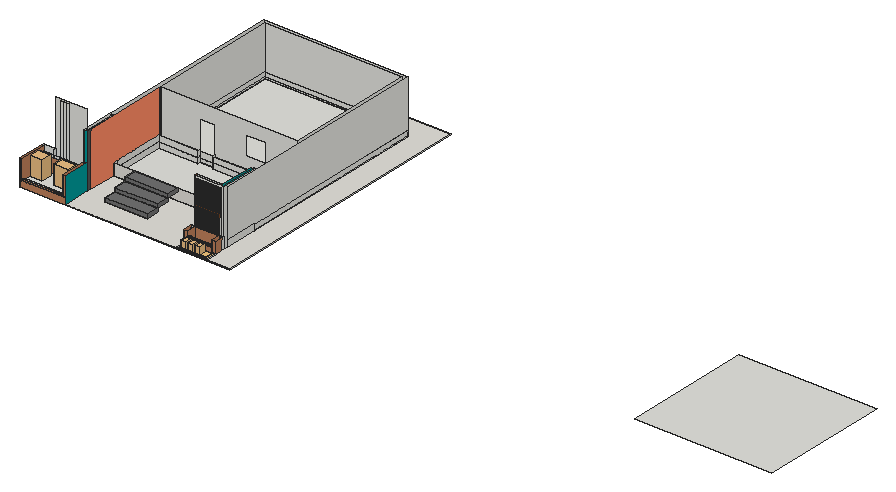
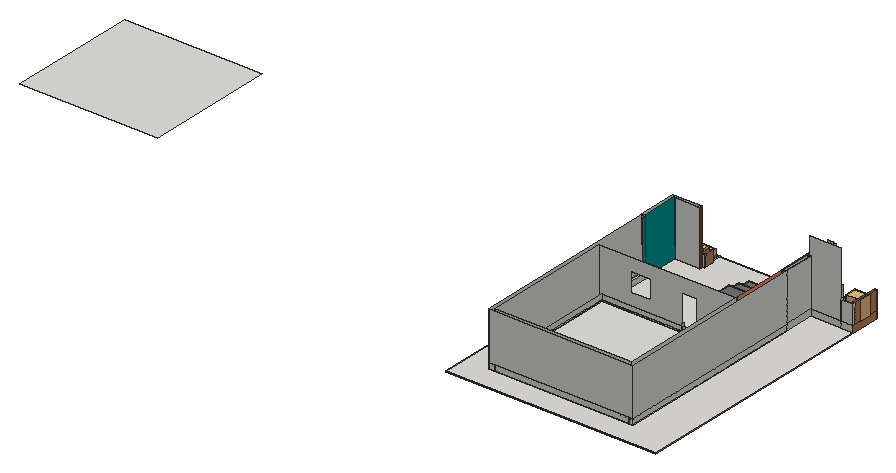
# SketchUp Ruby script. Lengths in inches.
U = 1.inch
M = Sketchup.active_model
def pt(a) = Geom::Point3d.new(a.map { |v| v * U })
def face(e, loops, mat)
  f = e.add_face(loops[0].map { |a| pt(a) })
  loops[1..].each { |l| e.add_face(l.map { |a| pt(a) }).erase! }
  f.material = f.back_material = mat if mat
  f
end
# faces: each face lists its corners as indices into pts; further lists are holes
def faces(e, pts, list, mat = nil) = list.each { |f| face(e, (f[0].is_a?(Array) ? f : [f]).map { |l| l.map { |i| pts[i] } }, mat) }
# xy, xz, yz: faces in a plane at the given z, y or x. An outline is a flat list of corners, or four numbers for a rectangle; further outlines are holes
def ring(l) = l.size == 4 ? [[l[0], l[1]], [l[2], l[1]], [l[2], l[3]], [l[0], l[3]]] : l.each_slice(2).to_a
def flat(e, list, mat, &to3) = list.each { |f| face(e, (f[0].is_a?(Array) ? f : [f]).map { |l| ring(l).map { |u, v| to3.(u, v) } }, mat) }
def xy(e, z, list, mat = nil) = flat(e, list, mat) { |x, y| [x, y, z] }
def xz(e, y, list, mat = nil) = flat(e, list, mat) { |x, z| [x, y, z] }
def yz(e, x, list, mat = nil) = flat(e, list, mat) { |y, z| [x, y, z] }
def lines(e, pts, list) = list.each { |a, b| e.add_line(pt(pts[a]), pt(pts[b])) }
# prism: a flat outline (further loops are holes) pulled along v
def prism(e, loops, v, mat = nil)
  f = face(e, loops, mat); d = Geom::Vector3d.new(v.map { |x| x * U })
  f.pushpull(f.normal.samedirection?(d) ? d.length : -d.length)
end
def box(e, o, s, mat = nil) = prism(e, [[o, [o[0] + s[0], o[1], o[2]], [o[0] + s[0], o[1] + s[1], o[2]], [o[0], o[1] + s[1], o[2]]]], [0, 0, s[2]], mat)
def at(x, y, z, deg = 0) = Geom::Transformation.translation(pt([x, y, z])) * Geom::Transformation.rotation(ORIGIN, Z_AXIS, deg.degrees)
def axes(o, x, y, z) = Geom::Transformation.new([*x, 0, *y, 0, *z, 0, *pt(o).to_a, 1])
def part(name) = M.definitions.add(name)
# library, detail: a bought-in or finely detailed component or shape, given as its bounding box
def library(name, o, s) = part(name).tap { |d| box(d.entities, o, s) }
def detail(e, o, s) = box(e.add_group.entities, o, s)
def put(e, d, t, mat = nil) = e.add_instance(d, t).tap { |i| i.material = mat if mat }
def group(e, t, mat = nil) = e.add_group.tap { |g| g.transformation = t; g.material = mat if mat }.entities
root = M.entities
M.materials.add("[Color B03]").color = [255, 140, 101]
M.materials.add("[Color H07]").color = [0, 153, 153]
M.materials.add("[Color M05]").color = [114, 114, 114]
M.materials.add("[Color M06]").color = [86, 86, 86]
M.materials.add("[Marble Carrara Gold Floor Tile]").color = [225, 223, 217]
M.materials.add("[Wood OSB]").color = [240, 195, 122]
M.materials.add("[Wood Veneer 01]").color = [120, 70, 37]
M.materials.add("[Wood Veneer 02]").color = [190, 128, 91]
c1 = library("Flower+vase",[-27.04,-0.0625,0],[7.8,7.11,11.89])
c2 = library("Decorative Plant",[-0.35,-0.24,0],[4.14,4.48,6.875])
xy(root,-18.75,[[114.76,294.58,448.89,619.58]])
xy(root,-14.75,[[[0,0,523.53,687.4],[104.7,148.58,464.7,628.58]]])
xy(root,-13.375,[[391.11,0,391.11,27.35,395.24,27.35,395.24,6.2,458.71,6.2,458.71,27.35,464.58,27.35,464.58,0],[386.33,27.35,395.89,48.85],[395.89,27.35,455.01,32.63],[455.01,27.35,464.58,48.85],[395.89,32.63,455.01,48.85],
  [386.33,48.85,464.58,53.1],[104.7,148.58,104.7,628.58,114.76,628.58,114.76,148.89,113.7,148.89,113.7,148.58],[113.7,148.58,114.76,148.89],[114.76,148.58,448.89,148.89],[448.89,148.58,455.7,148.89],
  [455.7,148.58,455.7,148.89,448.89,148.89,448.89,626.64,464.7,626.64,464.7,148.58],[448.89,626.64,464.7,628.58],[104.7,628.58,448.89,628.89]])
xy(root,-13.375,[[112.66,0,391.11,0,391.11,27.35,386.33,27.35,386.33,53.1,464.58,53.1,464.58,0,523.53,0,523.53,687.4,0,687.4,0,73.72,104.7,73.72,104.7,628.89,448.89,628.89,448.89,628.58,464.7,628.58,464.7,65.3,455.7,65.3,455.7,148.58,113.7,148.58,113.7,78.01,113.42,78.01,113.42,67.32,112.66,67.32]],"[Marble Carrara Gold Floor Tile]")
xy(root,-13.375,[[395.24,6.2,458.71,27.35]],"[Wood OSB]")
xy(root,-13.25,[[113.7,148.89,113.7,288.58,212.89,288.58,212.89,294.58,248.89,294.58,248.89,288.58,455.7,288.58,455.7,148.89]])
xy(root,-11.375,[[391.11,0,464.58,0,464.58,27.35,458.71,27.35,458.71,6.2,395.24,6.2,395.24,27.35,391.11,27.35]],"[Wood OSB]")
xy(root,-3.625,[[114.76,294.58,448.89,619.58]])
xy(root,-1.375,[[395.89,27.35,455.01,32.63]],"[Color M05]")
xy(root,0,[[1526.25,8.36,1868.25,333.36],[104.7,148.58,113.7,148.58,113.7,288.58,114.76,288.58,114.76,294.58,113.7,294.58,113.7,619.58,114.76,619.58,114.76,628.58,104.7,628.58],[113.7,148.58,114.76,288.58],[448.89,148.58,455.7,288.58],[455.7,148.58,464.7,148.58,464.7,626.64,448.89,626.64,448.89,619.58,455.7,619.58,455.7,294.58,448.89,294.58,448.89,288.58,455.7,288.58],
  [114.76,288.58,212.89,294.58],[248.89,288.58,448.89,294.58],[113.7,294.58,114.76,619.58],[448.89,294.58,455.7,619.58],[114.76,619.58,448.89,628.58],
  [448.89,626.64,464.7,628.58],[104.7,628.58,448.89,628.89]])
xy(root,2,[[0,0,4.34,67.36],[4.34,0,104.79,4.19],[4.34,4.19,104.79,57.44],[4.34,57.44,4.34,67.36,29.5,67.36,29.5,66.64,47.91,66.64,47.91,63.64,52.61,63.64,52.61,66.64,55.29,66.64,55.29,63.64,59.98,63.64,59.98,66.64,63.1,66.64,63.1,63.64,67.79,63.64,67.79,66.64,104.7,66.64,104.7,67.36,104.79,67.36,104.79,57.44],[47.91,63.64,52.61,66.64],
  [55.29,63.64,59.98,66.64],[63.1,63.64,67.79,66.64],[455.7,65.3,464.7,148.58],[29.5,66.64,104.7,67.36],[0,67.36,29.5,73.72],
  [29.5,67.36,104.7,73.72],[104.7,67.36,104.79,73.72],[104.7,73.72,104.7,148.58,110.64,148.58,110.64,78.01,104.79,78.01,104.79,73.72],[104.79,73.72,110.64,78.01]])
xz(root,0,[[391.11,-13.375,464.58,-11.375]])
xz(root,0,[[0,-14.75,523.53,-14.75,523.53,-13.375,112.66,-13.375,112.66,2,0,2],[0,2,4.34,50],[4.34,2,104.79,5.125],[104.79,2,112.66,50]],"[Wood Veneer 02]")
xz(root,4.19,[[4.34,2,104.79,5.125]])
xz(root,6.2,[[395.24,-13.375,458.71,-11.375]])
xz(root,27.35,[[391.11,-13.375,395.24,-11.375],[458.71,-13.375,464.58,-11.375]])
xz(root,27.35,[[386.33,-13.375,391.11,-13.375,391.11,-11.375,395.24,-11.375,395.24,-13.375,395.89,-13.375,395.89,14.625,386.33,14.625],[395.89,-13.375,455.01,-1.375],[455.01,-13.375,458.71,-13.375,458.71,-11.375,464.58,-11.375,464.58,14.91,455.01,14.91]],"[Wood Veneer 02]")
xz(root,32.63,[[395.89,-13.375,455.01,-1.375]])
xz(root,48.85,[[386.33,-13.375,395.89,14.625],[455.01,-13.375,464.58,14.6875]])
xz(root,48.85,[[395.89,-13.375,455.01,14.6875]],"[Wood Veneer 02]")
xz(root,53.1,[[386.33,-13.375,464.58,14.6875]])
xz(root,57.44,[[4.34,2,104.79,38.8125]],"[Wood Veneer 02]")
xz(root,63.64,[[47.91,2,52.61,38.8125],[55.29,2,59.98,38.8125],[63.1,2,67.79,38.8125]])
xz(root,65.3,[[455.7,-13.375,464.7,2],[455.7,2,464.7,120]])
xz(root,66.64,[[29.5,2,47.91,38.8125],[47.91,2,52.61,165.75],[52.61,2,55.29,38.8125],[55.29,2,59.98,165.75],[59.98,2,63.1,38.8125],
  [63.1,2,67.79,165.75],[67.79,2,104.7,38.8125]])
xz(root,67.32,[[112.66,-13.375,113.42,2],[104.79,2,112.66,50]])
xz(root,67.32,[[112.66,2,113.42,2,113.42,121.125,104.79,121.125,104.79,50,112.66,50]],"[Color H07]")
xz(root,67.36,[[0,2,4.34,50],[4.34,2,29.5,38.8125],[104.7,2,104.79,38.8125]])
xz(root,73.72,[[0,-13.375,29.5,2],[29.5,-13.375,104.7,2],[0,2,29.5,50],[29.5,2,29.5,165.75,106.01,165.75,106.01,120,104.7,120,104.7,2],[104.7,2,110.64,120]])
xz(root,78.01,[[113.42,-13.375,113.7,2],[104.79,2,110.64,107.35],[110.64,2,113.42,107.35],[113.42,2,113.7,2,113.7,120,110.64,120,110.64,107.35,113.42,107.35]])
xz(root,148.58,[[104.7,-14.75,113.7,-13.375],[113.7,-14.75,455.7,-13.375],[455.7,-14.75,464.7,-13.375],[104.7,-13.375,113.7,0],[113.7,-13.375,114.76,0],
  [448.89,-13.375,455.7,0],[455.7,-13.375,464.7,0],[104.7,0,113.7,2],[455.7,0,464.7,2],[104.7,2,110.64,120]])
xz(root,148.58,[[114.76,-13.375,448.89,-13.375,448.89,0,455.7,0,455.7,15,113.7,15,113.7,0,114.76,0]],"[Marble Carrara Gold Floor Tile]")
xz(root,148.89,[[113.7,-13.375,455.7,-13.25],[113.7,-13.25,455.7,-0.3125]])
xz(root,288.58,[[113.7,-13.25,212.89,0],[248.89,-13.25,455.7,0],[113.7,0,212.89,15],[248.89,0,455.7,15]])
xz(root,294.58,[[114.76,-18.75,212.89,-3.625],[212.89,-18.75,248.89,-13.25],[248.89,-18.75,448.89,-3.625],[212.89,-13.25,248.89,-3.625],[114.76,-3.625,212.89,0],
  [212.89,-3.625,248.89,11.625],[248.89,-3.625,448.89,0],[[113.7,0,113.7,120,455.7,120,455.7,0,448.89,0,448.89,11.625,248.89,11.625,248.89,84,212.89,84,212.89,11.625,114.76,11.625,114.76,0],[327.66,41.07,375.66,89.07]],[114.76,0,212.89,11.625],[248.89,0,448.89,11.625]])
xz(root,619.58,[[114.76,-18.75,448.89,-3.625],[114.76,-3.625,448.89,0],[113.7,0,114.76,0,114.76,11.625,448.89,11.625,448.89,0,455.7,0,455.7,120,113.7,120],[114.76,0,448.89,11.625]])
xz(root,626.64,[[448.89,-13.375,464.7,0]])
xz(root,628.58,[[104.7,-14.75,464.7,-13.375],[104.7,-13.375,114.76,0],[114.76,-13.375,448.89,0],[448.89,-13.375,464.7,0],[104.7,0,464.7,120]])
xz(root,628.89,[[104.7,-13.375,448.89,0]])
xz(root,687.4,[[0,-14.75,523.53,-13.375]])
yz(root,0,[[67.36,2,73.72,50]])
yz(root,0,[[0,-14.75,0,2,73.72,2,73.72,-13.375,687.4,-13.375,687.4,-14.75],[0,2,67.36,50]],"[Wood Veneer 02]")
yz(root,4.34,[[0,2,4.19,5.125],[57.44,2,67.36,38.8125]])
yz(root,4.34,[[4.19,2,57.44,2,57.44,38.8125,67.36,38.8125,67.36,50,0,50,0,5.125,4.19,5.125]],"[Wood Veneer 02]")
yz(root,29.5,[[66.64,2,67.36,38.8125],[67.36,2,73.72,50]])
yz(root,47.91,[[63.64,2,66.64,38.8125]])
yz(root,52.61,[[63.64,2,66.64,38.8125]])
yz(root,55.29,[[63.64,2,66.64,38.8125]])
yz(root,59.98,[[63.64,2,66.64,38.8125]])
yz(root,63.1,[[63.64,2,66.64,38.8125]])
yz(root,67.79,[[63.64,2,66.64,38.8125]])
yz(root,104.7,[[148.58,-14.75,628.58,-13.375],[73.72,-13.375,148.58,2],[148.58,-13.375,628.58,0],[628.58,-13.375,628.89,0],[148.58,0,628.58,120],
  [66.64,2,67.36,38.8125],[67.36,2,73.72,2,73.72,120,66.64,120,66.64,38.8125,67.36,38.8125],[73.72,2,148.58,120]])
yz(root,104.79,[[0,2,4.19,5.125],[57.44,2,67.32,38.8125],[67.32,2,67.36,38.8125],[67.36,2,67.36,38.8125,67.32,38.8125,67.32,121.125,152.44,121.125,152.44,107.35,78.01,107.35,78.01,2]])
yz(root,104.79,[[4.19,2,4.19,5.125,0,5.125,0,50,67.32,50,67.32,38.8125,57.44,38.8125,57.44,2]],"[Wood Veneer 02]")
yz(root,110.64,[[73.72,2,78.01,120],[78.01,2,148.58,120]])
yz(root,112.66,[[0,-13.375,67.32,50]],"[Color H07]")
yz(root,113.42,[[67.32,-13.375,78.01,-13.375,78.01,107.35,152.44,107.35,152.44,121.125,67.32,121.125]],"[Color M06]")
yz(root,113.7,[[148.58,-13.375,148.89,-0.3125],[148.89,-13.25,148.89,-0.3125,148.58,-0.3125,148.58,0,157.58,0,157.58,-13.25],[157.58,-13.25,288.58,0],[148.58,0,157.58,15],[157.58,0,288.58,15],
  [294.58,0,619.58,120]])
yz(root,113.7,[[78.01,-13.375,148.58,-13.375,148.58,15,288.58,15,288.58,120,78.01,120]],"[Color B03]")
yz(root,114.76,[[294.58,-18.75,619.58,-13.375],[148.58,-13.375,294.58,0],[294.58,-13.375,619.58,-3.625],[619.58,-13.375,628.58,0],[294.58,-3.625,619.58,0],
  [294.58,0,619.58,11.625]])
yz(root,212.89,[[288.58,-13.25,294.58,0],[288.58,0,294.58,15]])
yz(root,248.89,[[288.58,-13.25,294.58,0],[288.58,0,294.58,15]])
yz(root,386.33,[[27.35,-13.375,48.85,14.625],[48.85,-13.375,53.1,14.6875]],"[Wood Veneer 02]")
yz(root,390.38,[[60.8125,-13.625,54.8125,-13.53,56.92,118.16,57.01,124.36,57.02,124.46,63.01,124.36]],"[Wood Veneer 01]")
yz(root,391.11,[[0,-13.375,27.35,-11.375]])
yz(root,392.875,[[56.375,-13.55,58.48,118.13,56.92,118.16,54.8125,-13.53]],"[Wood Veneer 01]")
yz(root,395.24,[[6.2,-13.375,27.35,-11.375]])
yz(root,395.375,[[56.625,2.07,53.625,2.12,55.48,118.18,56.92,118.16,58.48,118.13]],"[Wood Veneer 01]")
yz(root,395.89,[[27.35,-13.375,32.63,-1.375],[28.97,0.13,28.61,0.18,28.28,0.32,28,0.53,27.78,0.82,27.64,1.15,27.59,1.51,27.64,1.86,27.78,2.19,28,2.48,28.28,2.7,28.61,2.84,28.97,2.88,29.32,2.84,29.66,2.7,29.94,2.48,30.16,2.19,30.3,1.86,30.34,1.51,30.3,1.15,30.16,0.82,29.94,0.53,29.66,0.32,29.32,0.18]])
yz(root,395.89,[[[32.63,-13.375,48.85,-13.375,48.85,14.625,27.35,14.625,27.35,-1.375,32.63,-1.375],[28.97,11.57,28.61,11.62,28.28,11.75,28,11.97,27.78,12.26,27.64,12.59,27.59,12.94,27.64,13.3,27.78,13.63,28,13.92,28.28,14.14,28.61,14.27,28.97,14.32,29.32,14.27,29.66,14.14,29.94,13.92,30.16,13.63,30.3,13.3,30.34,12.94,30.3,12.59,30.16,12.26,29.94,11.97,29.66,11.75,29.32,11.62],[28.97,7.19,28.61,7.24,28.28,7.38,28,7.6,27.78,7.88,27.64,8.21,27.59,8.57,27.64,8.93,27.78,9.26,28,9.54,28.28,9.76,28.61,9.9,28.97,9.94,29.32,9.9,29.66,9.76,29.94,9.54,30.16,9.26,30.3,8.93,30.34,8.57,30.3,8.21,30.16,7.88,29.94,7.6,29.66,7.38,29.32,7.24],[28.97,3.38,28.61,3.43,28.28,3.57,28,3.78,27.78,4.07,27.64,4.4,27.59,4.76,27.64,5.11,27.78,5.44,28,5.73,28.28,5.95,28.61,6.09,28.97,6.13,29.32,6.09,29.66,5.95,29.94,5.73,30.16,5.44,30.3,5.11,30.34,4.76,30.3,4.4,30.16,4.07,29.94,3.78,29.66,3.57,29.32,3.43],[28.97,0.13,28.61,0.18,28.28,0.32,28,0.53,27.78,0.82,27.64,1.15,27.59,1.51,27.64,1.86,27.78,2.19,28,2.48,28.28,2.7,28.61,2.84,28.97,2.88,29.32,2.84,29.66,2.7,29.94,2.48,30.16,2.19,30.3,1.86,30.34,1.51,30.3,1.15,30.16,0.82,29.94,0.53,29.66,0.32,29.32,0.18]]],"[Wood Veneer 02]")
yz(root,397.875,[[56.625,2.07,58.48,118.13,56.92,118.16,55.48,118.18,53.625,2.12]],"[Wood Veneer 01]")
yz(root,400.375,[[56.625,2.07,53.625,2.12,55.48,118.18,56.92,118.16,58.48,118.13]],"[Wood Veneer 01]")
yz(root,402.875,[[56.625,2.07,58.48,118.13,56.92,118.16,55.48,118.18,53.625,2.12]],"[Wood Veneer 01]")
yz(root,405.375,[[56.625,2.07,53.625,2.12,55.48,118.18,56.92,118.16,58.48,118.13]],"[Wood Veneer 01]")
yz(root,407.875,[[56.625,2.07,58.48,118.13,56.92,118.16,55.48,118.18,53.625,2.12]],"[Wood Veneer 01]")
yz(root,410.375,[[56.625,2.07,53.625,2.12,55.48,118.18,56.92,118.16,58.48,118.13]],"[Wood Veneer 01]")
yz(root,412.875,[[56.625,2.07,58.48,118.13,56.92,118.16,55.48,118.18,53.625,2.12]],"[Wood Veneer 01]")
yz(root,415.375,[[56.625,2.07,53.625,2.12,55.48,118.18,56.92,118.16,58.48,118.13]],"[Wood Veneer 01]")
yz(root,417.875,[[56.625,2.07,58.48,118.13,56.92,118.16,55.48,118.18,53.625,2.12]],"[Wood Veneer 01]")
yz(root,420.375,[[56.625,2.07,53.625,2.12,55.48,118.18,56.92,118.16,58.48,118.13]],"[Wood Veneer 01]")
yz(root,422.875,[[56.625,2.07,58.48,118.13,56.92,118.16,55.48,118.18,53.625,2.12]],"[Wood Veneer 01]")
yz(root,425.375,[[56.625,2.07,53.625,2.12,55.48,118.18,56.92,118.16,58.48,118.13]],"[Wood Veneer 01]")
yz(root,427.875,[[56.625,2.07,58.48,118.13,56.92,118.16,55.48,118.18,53.625,2.12]],"[Wood Veneer 01]")
yz(root,430.375,[[56.625,2.07,53.625,2.12,55.48,118.18,56.92,118.16,58.48,118.13]],"[Wood Veneer 01]")
yz(root,432.875,[[56.625,2.07,58.48,118.13,56.92,118.16,55.48,118.18,53.625,2.12]],"[Wood Veneer 01]")
yz(root,435.375,[[56.625,2.07,53.625,2.12,55.48,118.18,56.92,118.16,58.48,118.13]],"[Wood Veneer 01]")
yz(root,437.875,[[56.625,2.07,58.48,118.13,56.92,118.16,55.48,118.18,53.625,2.12]],"[Wood Veneer 01]")
yz(root,440.375,[[56.625,2.07,53.625,2.12,55.48,118.18,56.92,118.16,58.48,118.13]],"[Wood Veneer 01]")
yz(root,442.875,[[56.625,2.07,58.48,118.13,56.92,118.16,55.48,118.18,53.625,2.12]],"[Wood Veneer 01]")
yz(root,445.375,[[56.625,2.07,53.625,2.12,55.48,118.18,56.92,118.16,58.48,118.13]],"[Wood Veneer 01]")
yz(root,447.875,[[56.625,2.07,58.48,118.13,56.92,118.16,55.48,118.18,53.625,2.12]],"[Wood Veneer 01]")
yz(root,448.89,[[294.58,-18.75,619.58,-13.375],[148.58,-13.375,294.58,0],[294.58,-13.375,619.58,-3.625],[619.58,-13.375,626.64,0],[626.64,-13.375,628.58,0],
  [628.58,-13.375,628.89,0],[294.58,-3.625,619.58,0],[294.58,0,619.58,11.625]])
yz(root,450.375,[[56.625,2.07,53.625,2.12,55.48,118.18,56.92,118.16,58.48,118.13]],"[Wood Veneer 01]")
yz(root,452.875,[[56.625,2.07,58.48,118.13,56.92,118.16,55.48,118.18,53.625,2.12]],"[Wood Veneer 01]")
yz(root,454.76,[[60.81,-13.87,56.37,-13.8,56.375,-13.55,60.8125,-13.625],[56.37,-13.8,54.81,-13.78,56.92,118.16,58.48,118.13,56.375,-13.55]])
yz(root,454.76,[[148.86,-15.28,60.81,-13.87,60.8125,-13.625,63.01,124.36,151.07,122.96]],"[Color H07]")
yz(root,455.01,[[27.35,-13.375,32.63,-1.375]])
yz(root,455.01,[[[32.63,-13.375,32.63,-1.375,27.35,-1.375,27.35,14.91,48.85,14.91,48.85,-13.375],[28.97,11.57,29.32,11.62,29.66,11.75,29.94,11.97,30.16,12.26,30.3,12.59,30.34,12.94,30.3,13.3,30.16,13.63,29.94,13.92,29.66,14.14,29.32,14.27,28.97,14.32,28.61,14.27,28.28,14.14,28,13.92,27.78,13.63,27.64,13.3,27.59,12.94,27.64,12.59,27.78,12.26,28,11.97,28.28,11.75,28.61,11.62],[28.97,0.13,29.32,0.18,29.66,0.32,29.94,0.53,30.16,0.82,30.3,1.15,30.34,1.51,30.3,1.86,30.16,2.19,29.94,2.48,29.66,2.7,29.32,2.84,28.97,2.88,28.61,2.84,28.28,2.7,28,2.48,27.78,2.19,27.64,1.86,27.59,1.51,27.64,1.15,27.78,0.82,28,0.53,28.28,0.32,28.61,0.18]]],"[Wood Veneer 02]")
yz(root,455.7,[[65.3,-13.375,148.58,2],[148.58,-13.375,148.89,-0.3125],[148.89,-13.25,157.58,-13.25,157.58,0,148.58,0,148.58,-0.3125,148.89,-0.3125],[157.58,-13.25,288.58,0],[148.58,0,157.58,15],
  [157.58,0,288.58,15],[294.58,0,619.58,120]])
yz(root,455.7,[[65.3,2,65.3,120,157.58,120,157.58,15,148.58,15,148.58,2]],"[Color H07]")
yz(root,458.71,[[6.2,-13.375,27.35,-11.375]])
yz(root,462.78,[[148.86,-15.28,151.07,122.96,63.01,124.36,57.02,124.46,57.01,124.36,54.81,-13.78]])
yz(root,464.58,[[0,-13.375,27.35,-11.375],[48.85,-13.375,53.1,14.6875]])
yz(root,464.58,[[27.35,-13.375,48.85,14.91]],"[Wood Veneer 02]")
yz(root,464.7,[[148.58,-14.75,628.58,-13.375],[65.3,-13.375,148.58,2],[148.58,-13.375,626.64,0],[626.64,-13.375,628.58,0],[148.58,0,628.58,0,628.58,120,65.3,120,65.3,2,148.58,2]])
yz(root,523.53,[[0,-14.75,687.4,-13.375]])
p = [[462.78,54.81,-13.78],[454.76,54.81,-13.78],[454.76,56.37,-13.8],[454.76,60.81,-13.87],[454.76,148.86,-15.28],[462.78,148.86,-15.28],
  [454.76,151.07,122.96],[462.78,151.07,122.96],[452.875,56.92,118.16],[454.76,56.92,118.16],[462.78,57.01,124.36],[454.76,57.01,124.36],
  [450.45,57.01,124.36],[390.38,57.01,124.36],[390.38,56.92,118.16],[392.875,56.92,118.16],[395.375,56.92,118.16],[397.875,56.92,118.16],
  [400.375,56.92,118.16],[402.875,56.92,118.16],[405.375,56.92,118.16],[407.875,56.92,118.16],[410.375,56.92,118.16],[412.875,56.92,118.16],
  [415.375,56.92,118.16],[417.875,56.92,118.16],[420.375,56.92,118.16],[422.875,56.92,118.16],[425.375,56.92,118.16],[427.875,56.92,118.16],
  [430.375,56.92,118.16],[432.875,56.92,118.16],[435.375,56.92,118.16],[437.875,56.92,118.16],[440.375,56.92,118.16],[442.875,56.92,118.16],
  [445.375,56.92,118.16],[447.875,56.92,118.16],[450.375,56.92,118.16],[450.45,56.92,118.16],[450.45,60.8125,-13.625],[450.45,56.375,-13.55],
  [450.375,56.375,-13.55],[447.875,56.375,-13.55],[445.375,56.375,-13.55],[442.875,56.375,-13.55],[440.375,56.375,-13.55],[437.875,56.375,-13.55],
  [435.375,56.375,-13.55],[432.875,56.375,-13.55],[430.375,56.375,-13.55],[427.875,56.375,-13.55],[425.375,56.375,-13.55],[422.875,56.375,-13.55],
  [420.375,56.375,-13.55],[417.875,56.375,-13.55],[415.375,56.375,-13.55],[412.875,56.375,-13.55],[410.375,56.375,-13.55],[407.875,56.375,-13.55],
  [405.375,56.375,-13.55],[402.875,56.375,-13.55],[400.375,56.375,-13.55],[397.875,56.375,-13.55],[395.375,56.375,-13.55],[392.875,56.375,-13.55],
  [392.875,54.8125,-13.53],[390.38,54.8125,-13.53],[390.38,60.8125,-13.625],[395.375,58.48,118.13],[392.875,58.48,118.13],[395.375,56.625,2.07],
  [397.875,56.625,2.07],[400.375,58.48,118.13],[397.875,58.48,118.13],[400.375,56.625,2.07],[402.875,56.625,2.07],[405.375,58.48,118.13],
  [402.875,58.48,118.13],[405.375,56.625,2.07],[407.875,56.625,2.07],[410.375,58.48,118.13],[407.875,58.48,118.13],[410.375,56.625,2.07],
  [412.875,56.625,2.07],[415.375,58.48,118.13],[412.875,58.48,118.13],[415.375,56.625,2.07],[417.875,56.625,2.07],[420.375,58.48,118.13],
  [417.875,58.48,118.13],[420.375,56.625,2.07],[422.875,56.625,2.07],[425.375,58.48,118.13],[422.875,58.48,118.13],[425.375,56.625,2.07],
  [427.875,56.625,2.07],[430.375,58.48,118.13],[427.875,58.48,118.13],[430.375,56.625,2.07],[432.875,56.625,2.07],[435.375,58.48,118.13],
  [432.875,58.48,118.13],[435.375,56.625,2.07],[437.875,56.625,2.07],[440.375,58.48,118.13],[437.875,58.48,118.13],[440.375,56.625,2.07],
  [442.875,56.625,2.07],[445.375,58.48,118.13],[442.875,58.48,118.13],[445.375,56.625,2.07],[447.875,56.625,2.07],[450.375,58.48,118.13],
  [447.875,58.48,118.13],[450.375,56.625,2.07],[454.76,60.8125,-13.625],[454.76,56.375,-13.55],[452.875,56.375,-13.55],[450.45,56.625,2.07],
  [452.875,56.625,2.07],[454.76,58.48,118.13],[452.875,58.48,118.13],[450.45,63.01,124.36],[390.38,63.01,124.36],[401.32,63.01,124.36],
  [454.76,63.01,124.36],[395.89,28.61,0.18],[395.89,28.97,0.13],[455.01,28.97,0.13],[455.01,28.61,0.18],[395.89,29.32,0.18],
  [455.01,29.32,0.18],[395.89,28.28,0.32],[455.01,28.28,0.32],[395.89,29.66,0.32],[455.01,29.66,0.32],[395.89,28,0.53],
  [455.01,28,0.53],[395.89,29.94,0.53],[455.01,29.94,0.53],[395.89,27.78,0.82],[455.01,27.78,0.82],[395.89,30.16,0.82],
  [455.01,30.16,0.82],[395.89,27.64,1.15],[455.01,27.64,1.15],[395.89,30.3,1.15],[455.01,30.3,1.15],[395.89,27.59,1.51],
  [455.01,27.59,1.51],[395.89,30.34,1.51],[455.01,30.34,1.51],[395.89,27.64,1.86],[455.01,27.64,1.86],[395.89,30.3,1.86],
  [455.01,30.3,1.86],[395.89,27.78,2.19],[455.01,27.78,2.19],[395.89,30.16,2.19],[455.01,30.16,2.19],[397.875,53.625,2.12],
  [395.375,53.625,2.12],[397.875,55.48,118.18],[395.375,55.48,118.18],[402.875,53.625,2.12],[400.375,53.625,2.12],[402.875,55.48,118.18],
  [400.375,55.48,118.18],[407.875,53.625,2.12],[405.375,53.625,2.12],[407.875,55.48,118.18],[405.375,55.48,118.18],[412.875,53.625,2.12],
  [410.375,53.625,2.12],[412.875,55.48,118.18],[410.375,55.48,118.18],[417.875,53.625,2.12],[415.375,53.625,2.12],[417.875,55.48,118.18],
  [415.375,55.48,118.18],[422.875,53.625,2.12],[420.375,53.625,2.12],[422.875,55.48,118.18],[420.375,55.48,118.18],[427.875,53.625,2.12],
  [425.375,53.625,2.12],[427.875,55.48,118.18],[425.375,55.48,118.18],[432.875,53.625,2.12],[430.375,53.625,2.12],[432.875,55.48,118.18],
  [430.375,55.48,118.18],[437.875,53.625,2.12],[435.375,53.625,2.12],[437.875,55.48,118.18],[435.375,55.48,118.18],[442.875,53.625,2.12],
  [440.375,53.625,2.12],[442.875,55.48,118.18],[440.375,55.48,118.18],[447.875,53.625,2.12],[445.375,53.625,2.12],[447.875,55.48,118.18],
  [445.375,55.48,118.18],[450.45,53.625,2.12],[450.375,53.625,2.12],[452.875,53.625,2.12],[450.45,55.48,118.18],[450.375,55.48,118.18],
  [452.875,55.48,118.18],[450.45,58.48,118.13],[395.89,28,2.48],[455.01,28,2.48],[395.89,29.94,2.48],[455.01,29.94,2.48],
  [395.89,28.28,2.7],[455.01,28.28,2.7],[395.89,29.66,2.7],[455.01,29.66,2.7],[395.89,28.61,2.84],[455.01,28.61,2.84],
  [395.89,29.32,2.84],[455.01,29.32,2.84],[395.89,28.97,2.88],[455.01,28.97,2.88],[390.375,56.625,2.07],[390.375,58.48,118.13]]
faces(root,p,[[0,1,2,3,4,5],[5,4,6,7],[8,9,1,0,10,11,12,13,14,15,16,17,18,19,20,21,22,23,24,25,26,27,28,29,30,31,32,33,34,35,36,37,38,39],[40,41,42,43,44,45,46,47,48,49,50,51,52,53,54,55,56,57,58,59,60,61,62,63,64,65,66,67,68],[72,71,64,63],[76,75,62,61],[80,79,60,59],[84,83,58,57],
  [88,87,56,55],[92,91,54,53],[96,95,52,51],[100,99,50,49],[104,103,48,47],[108,107,46,45],[112,111,44,43],[40,116,117,118,41],
  [119,115,42,41],[120,119,41,118],[123,40,68,124,125],[123,126,116,40],[71,72,161,162],[75,76,165,166],[79,80,169,170],[83,84,173,174],
  [87,88,177,178],[91,92,181,182],[95,96,185,186],[99,100,189,190],[103,104,193,194],[107,108,197,198],[111,112,201,202],[115,119,205,206],
  [119,120,207,205],[69,74,72,71],[73,78,76,75],[77,82,80,79],[81,86,84,83],[85,90,88,87],[89,94,92,91],[93,98,96,95],
  [97,102,100,99],[101,106,104,103],[105,110,108,107],[109,114,112,111],[113,211,122,120,119,115]])
faces(root,p,[[69,70,65,64,71],[73,74,72,63,62,75],[77,78,76,61,60,79],[81,82,80,59,58,83],[85,86,84,57,56,87],[89,90,88,55,54,91],[93,94,92,53,52,95],[97,98,96,51,50,99],
  [101,102,100,49,48,103],[105,106,104,47,46,107],[109,110,108,45,44,111],[113,114,112,43,42,115],[121,122,120,118,117],[14,67,66,15],[163,164,162,161],[167,168,166,165],
  [171,172,170,169],[175,176,174,173],[179,180,178,177],[183,184,182,181],[187,188,186,185],[191,192,190,189],[195,196,194,193],[199,200,198,197],
  [203,204,202,201],[208,209,206,205,207,210]],"[Wood Veneer 01]")
faces(root,p,[[127,128,129,130],[128,131,132,129],[133,127,130,134],[131,135,136,132],[137,133,134,138],[135,139,140,136],[141,137,138,142],[139,143,144,140],
  [145,141,142,146],[143,147,148,144],[149,145,146,150],[147,151,152,148],[153,149,150,154],[151,155,156,152],[157,153,154,158],[155,159,160,156],
  [212,157,158,213],[159,214,215,160],[216,212,213,217],[214,218,219,215],[220,216,217,221],[218,222,223,219],[224,220,221,225],[222,224,225,223]],"[Color M05]")
lines(root,p,[[226,227]])
put(root,c1,axes([438.09,5.58,-13.375],[1.518,0,0],[0,2.277,0],[0,0,1.518]))
put(root,c1,axes([454.4,5.58,-13.375],[1.518,0,0],[0,2.277,0],[0,0,1.518]))
put(root,c1,axes([472.02,5.58,-13.375],[1.518,0,0],[0,2.277,0],[0,0,1.518]))
g1 = group(root,at(177.07,12.71,2),"[Color M05]")
xy(g1,-14,[[-9.96,42.3,96.98,73.49]])
xy(g1,-5,[[-9.96,42.3,96.98,73.49],[-9.96,73.49,96.98,104.68]])
xy(g1,4,[[-9.96,73.49,96.98,104.68],[-9.96,104.68,96.98,135.86]])
xy(g1,13,[[-9.96,104.68,96.98,135.86]])
xz(g1,42.3,[[-9.96,-14,96.98,-5]])
xz(g1,73.49,[[-9.96,-14,96.98,-5],[-9.96,-5,96.98,4]])
xz(g1,104.68,[[-9.96,-5,96.98,4],[-9.96,4,96.98,13]])
xz(g1,135.86,[[-9.96,4,96.98,13]])
yz(g1,-9.96,[[42.3,-14,73.49,-5],[73.49,-5,104.68,4],[104.68,4,135.86,13]])
yz(g1,96.98,[[42.3,-14,73.49,-5],[73.49,-5,104.68,4],[104.68,4,135.86,13]])
put(root,c2,axes([66.85,24.99,2],[8.95467,0,0],[0,5.84118,0],[0,0,6.80394]))
put(root,c2,axes([1.1,24.99,2],[8.95467,0,0],[0,5.84118,0],[0,0,6.80394]))
